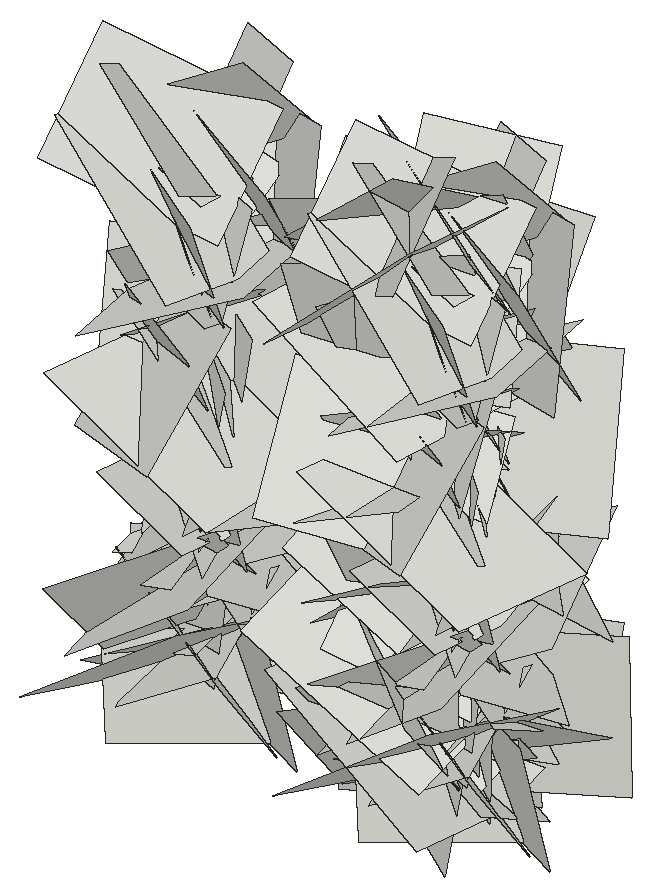
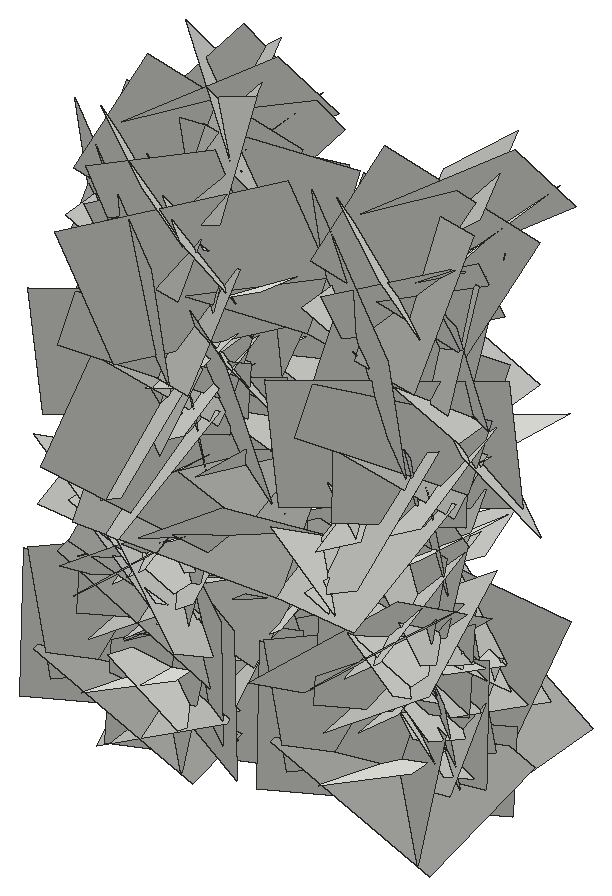
# SketchUp Ruby script. Lengths in inches.
U = 1.inch
M = Sketchup.active_model
def pt(a) = Geom::Point3d.new(a.map { |v| v * U })
def face(e, loops, mat)
  f = e.add_face(loops[0].map { |a| pt(a) })
  loops[1..].each { |l| e.add_face(l.map { |a| pt(a) }).erase! }
  f.material = f.back_material = mat if mat
  f
end
# faces: each face lists its corners as indices into pts; further lists are holes
def faces(e, pts, list, mat = nil) = list.each { |f| face(e, (f[0].is_a?(Array) ? f : [f]).map { |l| l.map { |i| pts[i] } }, mat) }
# xy, xz, yz: faces in a plane at the given z, y or x. An outline is a flat list of corners, or four numbers for a rectangle; further outlines are holes
def ring(l) = l.size == 4 ? [[l[0], l[1]], [l[2], l[1]], [l[2], l[3]], [l[0], l[3]]] : l.each_slice(2).to_a
def flat(e, list, mat, &to3) = list.each { |f| face(e, (f[0].is_a?(Array) ? f : [f]).map { |l| ring(l).map { |u, v| to3.(u, v) } }, mat) }
def xy(e, z, list, mat = nil) = flat(e, list, mat) { |x, y| [x, y, z] }
def xz(e, y, list, mat = nil) = flat(e, list, mat) { |x, z| [x, y, z] }
def yz(e, x, list, mat = nil) = flat(e, list, mat) { |y, z| [x, y, z] }
def lines(e, pts, list) = list.each { |a, b| e.add_line(pt(pts[a]), pt(pts[b])) }
# prism: a flat outline (further loops are holes) pulled along v
def prism(e, loops, v, mat = nil)
  f = face(e, loops, mat); d = Geom::Vector3d.new(v.map { |x| x * U })
  f.pushpull(f.normal.samedirection?(d) ? d.length : -d.length)
end
def box(e, o, s, mat = nil) = prism(e, [[o, [o[0] + s[0], o[1], o[2]], [o[0] + s[0], o[1] + s[1], o[2]], [o[0], o[1] + s[1], o[2]]]], [0, 0, s[2]], mat)
def at(x, y, z, deg = 0) = Geom::Transformation.translation(pt([x, y, z])) * Geom::Transformation.rotation(ORIGIN, Z_AXIS, deg.degrees)
def axes(o, x, y, z) = Geom::Transformation.new([*x, 0, *y, 0, *z, 0, *pt(o).to_a, 1])
def part(name) = M.definitions.add(name)
# library, detail: a bought-in or finely detailed component or shape, given as its bounding box
def library(name, o, s) = part(name).tap { |d| box(d.entities, o, s) }
def detail(e, o, s) = box(e.add_group.entities, o, s)
def put(e, d, t, mat = nil) = e.add_instance(d, t).tap { |i| i.material = mat if mat }
def group(e, t, mat = nil) = e.add_group.tap { |g| g.transformation = t; g.material = mat if mat }.entities
root = M.entities
c1 = part("Component\#6")
p = [[0.01,0,0],[0,3.24,4.54],[4.32,3.24,4.54],[4.33,0,0]]
faces(c1.entities,p,[[0,1,2,3]])
put(root,c1,axes([38.11,169.73,5.36],[-0.07377,0.11031,-0.61615],[-0.06228,-0.61836,-0.10407],[-0.66058,0.04598,0.07863]))
put(root,c1,axes([28.31,170.45,6.95],[0.13562,-0.59571,0.16409],[-0.06684,0.15411,0.60864],[-0.65155,-0.13981,-0.02828]))
put(root,c1,axes([34.14,170.45,6.95],[-0.13562,-0.59571,0.16409],[0.06684,0.15411,0.60864],[0.65155,-0.13981,-0.02828]))
put(root,c1,axes([38.11,170.45,6.95],[0.13562,-0.59571,0.16409],[-0.06684,0.15411,0.60864],[-0.65155,-0.13981,-0.02828]))
put(root,c1,axes([24.34,172.51,13.7],[-0.18405,-0.71312,-0.93832],[-0.0125,-0.94735,0.72216],[1.2492,-0.11455,-0.13102]))
put(root,c1,axes([38.11,172.51,13.7],[0.18405,-0.71312,-0.93832],[0.0125,-0.94735,0.72216],[-1.2492,-0.11455,-0.13102]))
put(root,c1,axes([34.14,172.51,13.7],[-0.18405,-0.71312,-0.93832],[-0.0125,-0.94735,0.72216],[1.2492,-0.11455,-0.13102]))
put(root,c1,axes([24.34,166.89,12.83],[0.13197,1.26874,-0.04114],[0.28106,-0.06642,-1.24587],[1.31589,-0.11305,0.27023]))
put(root,c1,axes([38.11,166.89,12.83],[-0.13197,1.26874,-0.04114],[-0.28106,-0.06642,-1.24587],[-1.31589,-0.11305,0.27023]))
put(root,c1,axes([34.14,166.89,12.83],[0.13197,1.26874,-0.04114],[0.28106,-0.06642,-1.24587],[1.31589,-0.11305,0.27023]))
put(root,c1,axes([28.31,170.4375,18.81],[0.19883,-0.70321,0.38228],[0.06935,0.40479,0.71252],[-0.84558,-0.13215,0.14832]))
put(root,c1,axes([34.14,170.4375,18.81],[-0.19883,-0.70321,0.38228],[-0.06935,0.40479,0.71252],[0.84558,-0.13215,0.14832]))
put(root,c1,axes([38.11,170.4375,18.81],[0.19883,-0.70321,0.38228],[0.06935,0.40479,0.71252],[-0.84558,-0.13215,0.14832]))
put(root,c1,axes([24.34,172.01,0.23],[-0.18306,-1.21621,0.26629],[-0.00588,0.26959,1.22768],[1.31971,-0.16751,0.04241]))
put(root,c1,axes([38.11,172.01,0.23],[0.18306,-1.21621,0.26629],[0.00588,0.26959,1.22768],[-1.31971,-0.16751,0.04241]))
put(root,c1,axes([34.14,172.01,0.23],[-0.18306,-1.21621,0.26629],[-0.00588,0.26959,1.22768],[1.31971,-0.16751,0.04241]))
put(root,c1,axes([24.34,167.43,21.54],[0.05686,1.16606,-0.16138],[-0.18622,-0.15181,-1.15529],[1.23383,-0.07665,-0.16693]))
put(root,c1,axes([38.11,167.43,21.54],[-0.05686,1.16606,-0.16138],[0.18622,-0.15181,-1.15529],[-1.23383,-0.07665,-0.16693]))
put(root,c1,axes([34.14,167.43,21.54],[0.05686,1.16606,-0.16138],[-0.18622,-0.15181,-1.15529],[1.23383,-0.07665,-0.16693]))
put(root,c1,axes([24.34,170.29,20.28],[0.01759,0.35165,-0.94572],[0.09141,-0.94289,-0.34909],[1.06561,0.07508,0.04555]))
put(root,c1,axes([38.11,170.29,20.28],[-0.01759,0.35165,-0.94572],[-0.09141,-0.94289,-0.34909],[-1.06561,0.07508,0.04555]))
put(root,c1,axes([34.14,170.29,20.28],[0.01759,0.35165,-0.94572],[0.09141,-0.94289,-0.34909],[1.06561,0.07508,0.04555]))
put(root,c1,axes([24.34,166.61,20.4],[0.01588,0.7114,0.79833],[-0.18087,0.78977,-0.70057],[1.11894,0.11757,-0.12458]))
put(root,c1,axes([38.11,166.61,20.4],[-0.01588,0.7114,0.79833],[0.18087,0.78977,-0.70057],[-1.11894,0.11757,-0.12458]))
put(root,c1,axes([34.14,166.61,20.4],[0.01588,0.7114,0.79833],[-0.18087,0.78977,-0.70057],[1.11894,0.11757,-0.12458]))
put(root,c1,axes([28.31,169.875,11.58],[0.08121,-0.31714,0.54408],[-0.11401,0.53345,0.32609],[-0.65774,-0.13162,0.01065]))
put(root,c1,axes([34.14,169.875,11.58],[-0.08121,-0.31714,0.54408],[0.11401,0.53345,0.32609],[0.65774,-0.13162,0.01065]))
put(root,c1,axes([38.11,169.875,11.58],[0.08121,-0.31714,0.54408],[-0.11401,0.53345,0.32609],[-0.65774,-0.13162,0.01065]))
put(root,c1,axes([24.34,169.82,1.95],[-0.02915,-0.64251,0.76006],[-0.08177,0.75943,0.6392],[1.05178,0.04123,0.07076]))
put(root,c1,axes([38.11,169.82,1.95],[0.02915,-0.64251,0.76006],[0.08177,0.75943,0.6392],[-1.05178,0.04123,0.07076]))
put(root,c1,axes([34.14,169.82,1.95],[-0.02915,-0.64251,0.76006],[-0.08177,0.75943,0.6392],[1.05178,0.04123,0.07076]))
put(root,c1,axes([24.34,173.1,4.27],[0.006,-1.20261,-0.38975],[-0.07836,-0.3894,1.20046],[1.33775,-0.01742,0.07206]))
put(root,c1,axes([38.11,173.1,4.27],[-0.006,-1.20261,-0.38975],[0.07836,-0.3894,1.20046],[-1.33775,-0.01742,0.07206]))
put(root,c1,axes([34.14,173.1,4.27],[0.006,-1.20261,-0.38975],[-0.07836,-0.3894,1.20046],[1.33775,-0.01742,0.07206]))
put(root,c1,axes([28.31,169.57,7.53],[-0.02893,-0.34038,0.60393],[0.06424,0.60091,0.34142],[-0.73203,0.06619,0.00609]))
put(root,c1,axes([34.14,169.57,7.53],[0.02893,-0.34038,0.60393],[-0.06424,0.60091,0.34142],[0.73203,0.06619,0.00609]))
put(root,c1,axes([38.11,169.57,7.53],[-0.02893,-0.34038,0.60393],[0.06424,0.60091,0.34142],[-0.73203,0.06619,0.00609]))
put(root,c1,axes([24.34,172.68,14.25],[0.15371,-1.16437,-0.05617],[0.14183,-0.0396,1.1664],[1.22751,0.15038,-0.12774]))
put(root,c1,axes([38.11,172.68,14.25],[-0.15371,-1.16437,-0.05617],[-0.14183,-0.0396,1.1664],[-1.22751,0.15038,-0.12774]))
put(root,c1,axes([34.14,172.68,14.25],[0.15371,-1.16437,-0.05617],[0.14183,-0.0396,1.1664],[1.22751,0.15038,-0.12774]))
put(root,c1,axes([28.31,172.08,18.68],[0.05145,-0.65016,0.07549],[-0.09383,0.06848,0.64671],[-0.68743,-0.05801,-0.08262]))
put(root,c1,axes([38.11,172.08,18.68],[0.05145,-0.65016,0.07549],[-0.09383,0.06848,0.64671],[-0.68743,-0.05801,-0.08262]))
put(root,c1,axes([34.14,172.08,18.68],[-0.05145,-0.65016,0.07549],[0.09383,0.06848,0.64671],[0.68743,-0.05801,-0.08262]))
put(root,c1,axes([28.31,168.08,6.15],[0.10311,0.69666,0.5447],[0.01855,0.54636,-0.70191],[-0.9372,0.08746,0.04604]))
put(root,c1,axes([34.14,168.08,6.15],[-0.10311,0.69666,0.5447],[-0.01855,0.54636,-0.70191],[0.9372,0.08746,0.04604]))
put(root,c1,axes([38.11,168.08,6.15],[0.10311,0.69666,0.5447],[0.01855,0.54636,-0.70191],[-0.9372,0.08746,0.04604]))
put(root,c1,axes([24.34,170.37,5.28],[-0.04044,0.69271,-0.86885],[0.14808,-0.85947,-0.69137],[1.16852,0.13289,0.05755]))
put(root,c1,axes([38.11,170.37,5.28],[0.04044,0.69271,-0.86885],[-0.14808,-0.85947,-0.69137],[-1.16852,0.13289,0.05755]))
put(root,c1,axes([34.14,170.37,5.28],[-0.04044,0.69271,-0.86885],[0.14808,-0.85947,-0.69137],[1.16852,0.13289,0.05755]))
put(root,c1,axes([24.34,171.61,19.65],[-0.05512,0.44879,-0.89687],[-0.12411,-0.89465,-0.44089],[1.05579,-0.08174,-0.09865]))
put(root,c1,axes([38.11,171.61,19.65],[0.05512,0.44879,-0.89687],[0.12411,-0.89465,-0.44089],[-1.05579,-0.08174,-0.09865]))
put(root,c1,axes([34.14,171.61,19.65],[-0.05512,0.44879,-0.89687],[-0.12411,-0.89465,-0.44089],[1.05579,-0.08174,-0.09865]))
put(root,c1,axes([24.34,172.8125,18.6875],[-0.10377,-0.25363,-0.96814],[0.17625,-0.96337,0.23557],[1.04612,0.13715,-0.13572]))
put(root,c1,axes([38.11,172.8125,18.6875],[0.10377,-0.25363,-0.96814],[-0.17625,-0.96337,0.23557],[-1.04612,0.13715,-0.13572]))
put(root,c1,axes([34.14,172.8125,18.6875],[-0.10377,-0.25363,-0.96814],[0.17625,-0.96337,0.23557],[1.04612,0.13715,-0.13572]))
put(root,c1,axes([24.34,173.43,2.26],[0.13173,-0.86629,-0.47025],[-0.00519,-0.47451,0.87284],[1.04483,0.10686,0.06363]))
put(root,c1,axes([38.11,173.43,2.26],[-0.13173,-0.86629,-0.47025],[0.00519,-0.47451,0.87284],[-1.04483,0.10686,0.06363]))
put(root,c1,axes([34.14,173.43,2.26],[0.13173,-0.86629,-0.47025],[-0.00519,-0.47451,0.87284],[1.04483,0.10686,0.06363]))
put(root,c1,axes([28.31,172.62,2.82],[0.11022,-0.07985,-0.84847],[-0.01268,-0.85481,0.07898],[-0.90326,0.00226,-0.10464]))
put(root,c1,axes([34.14,172.62,2.82],[-0.11022,-0.07985,-0.84847],[0.01268,-0.85481,0.07898],[0.90326,0.00226,-0.10464]))
put(root,c1,axes([38.11,172.62,2.82],[0.11022,-0.07985,-0.84847],[-0.01268,-0.85481,0.07898],[-0.90326,0.00226,-0.10464]))
put(root,c1,axes([38.11,172.18,10.26],[-0.13568,0.14362,-0.9313],[-0.0793,-0.93844,-0.13444],[-0.9957,0.05517,0.13761]))
put(root,c1,axes([24.34,172.18,10.26],[0.13568,0.14362,-0.9313],[0.0793,-0.93844,-0.13444],[0.9957,0.05517,0.13761]))
put(root,c1,axes([34.14,172.18,10.26],[0.13568,0.14362,-0.9313],[0.0793,-0.93844,-0.13444],[0.9957,0.05517,0.13761]))
put(root,c1,axes([28.31,169.25,3.37],[0.12984,0.58451,0.34416],[0.01188,0.34794,-0.59491],[-0.71891,0.11132,0.05233]))
put(root,c1,axes([34.14,169.25,3.37],[-0.12984,0.58451,0.34416],[-0.01188,0.34794,-0.59491],[0.71891,0.11132,0.05233]))
put(root,c1,axes([38.11,169.25,3.37],[0.12984,0.58451,0.34416],[0.01188,0.34794,-0.59491],[-0.71891,0.11132,0.05233]))
put(root,c1,axes([24.34,174.625,6.88],[0.07025,-1.10898,-0.49527],[-0.16839,-0.49966,1.09755],[1.27636,-0.00489,0.17206]))
put(root,c1,axes([38.11,174.625,6.88],[-0.07025,-1.10898,-0.49527],[0.16839,-0.49966,1.09755],[-1.27636,-0.00489,0.17206]))
put(root,c1,axes([34.14,174.625,6.88],[0.07025,-1.10898,-0.49527],[-0.16839,-0.49966,1.09755],[1.27636,-0.00489,0.17206]))
put(root,c1,axes([24.34,173.47,4.9],[0.07332,-0.2848,-0.87141],[-0.0336,-0.87411,0.28317],[0.9712,-0.00874,0.07558]))
put(root,c1,axes([38.11,173.47,4.9],[-0.07332,-0.2848,-0.87141],[0.0336,-0.87411,0.28317],[-0.9712,-0.00874,0.07558]))
put(root,c1,axes([34.14,173.47,4.9],[0.07332,-0.2848,-0.87141],[-0.0336,-0.87411,0.28317],[0.9712,-0.00874,0.07558]))
put(root,c1,axes([28.31,169.67,8.54],[0.12628,0.08221,0.86907],[0.11161,0.86937,-0.09667],[-0.91857,0.11693,0.10773]))
put(root,c1,axes([34.14,169.67,8.54],[-0.12628,0.08221,0.86907],[-0.11161,0.86937,-0.09667],[0.91857,0.11693,0.10773]))
put(root,c1,axes([38.11,169.67,8.54],[0.12628,0.08221,0.86907],[0.11161,0.86937,-0.09667],[-0.91857,0.11693,0.10773]))
put(root,c1,axes([28.31,173.61,18.42],[-0.00387,-0.64214,-0.38262],[-0.01033,-0.38255,0.64212],[-0.79227,0.00812,-0.0065]))
put(root,c1,axes([34.14,173.61,18.42],[0.00387,-0.64214,-0.38262],[0.01033,-0.38255,0.64212],[0.79227,0.00812,-0.0065]))
put(root,c1,axes([38.11,173.61,18.42],[-0.00387,-0.64214,-0.38262],[-0.01033,-0.38255,0.64212],[-0.79227,0.00812,-0.0065]))
put(root,c1,axes([24.34,173.47,6.03],[-0.02519,-0.71274,-0.22366],[0.1783,-0.22314,0.69319],[0.7715,0.02829,-0.1675]))
put(root,c1,axes([38.11,173.47,6.03],[0.02519,-0.71274,-0.22366],[-0.1783,-0.22314,0.69319],[-0.7715,0.02829,-0.1675]))
put(root,c1,axes([34.14,173.47,6.03],[-0.02519,-0.71274,-0.22366],[0.1783,-0.22314,0.69319],[0.7715,0.02829,-0.1675]))
put(root,c1,axes([24.34,170.23,14.27],[-0.02775,1.05616,-0.50439],[-0.01222,-0.50473,-1.05626],[1.24058,0.01865,-0.02169]))
put(root,c1,axes([38.11,170.23,14.27],[0.02775,1.05616,-0.50439],[0.01222,-0.50473,-1.05626],[-1.24058,0.01865,-0.02169]))
put(root,c1,axes([34.14,170.23,14.27],[-0.02775,1.05616,-0.50439],[-0.01222,-0.50473,-1.05626],[1.24058,0.01865,-0.02169]))
put(root,c1,axes([24.34,172.3,17.31],[-0.17712,-0.66279,0.75583],[0.05377,0.75967,0.67737],[1.06423,-0.14869,0.09157]))
put(root,c1,axes([38.11,172.3,17.31],[0.17712,-0.66279,0.75583],[-0.05377,0.75967,0.67737],[-1.06423,-0.14869,0.09157]))
put(root,c1,axes([34.14,172.3,17.31],[-0.17712,-0.66279,0.75583],[0.05377,0.75967,0.67737],[1.06423,-0.14869,0.09157]))
put(root,c1,axes([24.34,171.9,21.66],[0.05821,0.63814,-1.10333],[0.23209,-1.09266,-0.62107],[1.33097,0.16262,0.15656]))
put(root,c1,axes([38.11,171.9,21.66],[-0.05821,0.63814,-1.10333],[-0.23209,-1.09266,-0.62107],[-1.33097,0.16262,0.15656]))
put(root,c1,axes([34.14,171.9,21.66],[0.05821,0.63814,-1.10333],[0.23209,-1.09266,-0.62107],[1.33097,0.16262,0.15656]))
put(root,c1,axes([28.31,171.64,6.09],[0.04085,-0.22846,0.61977],[-0.06336,0.61707,0.23119],[-0.6973,-0.06945,0.0153]))
put(root,c1,axes([34.14,171.64,6.09],[-0.04085,-0.22846,0.61977],[0.06336,0.61707,0.23119],[0.6973,-0.06945,0.0153]))
put(root,c1,axes([38.11,171.64,6.09],[0.04085,-0.22846,0.61977],[-0.06336,0.61707,0.23119],[-0.6973,-0.06945,0.0153]))
put(root,c1,axes([24.34,170.14,10.52],[0.06349,0.95893,0.01002],[-0.03302,0.01198,-0.96028],[1.01599,-0.05954,-0.03183]))
put(root,c1,axes([38.11,170.14,10.52],[-0.06349,0.95893,0.01002],[0.03302,0.01198,-0.96028],[-1.01599,-0.05954,-0.03183]))
put(root,c1,axes([34.14,170.14,10.52],[0.06349,0.95893,0.01002],[-0.03302,0.01198,-0.96028],[1.01599,-0.05954,-0.03183]))
put(root,c1,axes([28.31,174.87,19.3],[0.1513,-0.51657,-0.73784],[0.06675,-0.7395,0.52991],[-0.9524,-0.13389,-0.08008]))
put(root,c1,axes([34.14,174.87,19.3],[-0.1513,-0.51657,-0.73784],[-0.06675,-0.7395,0.52991],[0.9524,-0.13389,-0.08008]))
put(root,c1,axes([38.11,174.87,19.3],[0.1513,-0.51657,-0.73784],[0.06675,-0.7395,0.52991],[-0.9524,-0.13389,-0.08008]))
put(root,c1,axes([24.34,172.92,11.6],[0.15777,-0.72106,0.34948],[-0.01112,0.35368,0.73418],[0.84929,0.13857,-0.05531]))
put(root,c1,axes([38.11,172.92,11.6],[-0.15777,-0.72106,0.34948],[0.01112,0.35368,0.73418],[-0.84929,0.13857,-0.05531]))
put(root,c1,axes([34.14,172.92,11.6],[0.15777,-0.72106,0.34948],[-0.01112,0.35368,0.73418],[0.84929,0.13857,-0.05531]))
put(root,c1,axes([24.34,169.35,10.4],[-0.15861,0.37048,1.309],[0.06067,1.31744,-0.36632],[1.44077,-0.01469,0.15953]))
put(root,c1,axes([38.11,169.35,10.4],[0.15861,0.37048,1.309],[-0.06067,1.31744,-0.36632],[-1.44077,-0.01469,0.15953]))
put(root,c1,axes([34.14,169.35,10.4],[-0.15861,0.37048,1.309],[0.06067,1.31744,-0.36632],[1.44077,-0.01469,0.15953]))
put(root,c1,axes([24.34,171.5,10.51],[0.09816,1.08592,-0.68794],[-0.27584,-0.65961,-1.07622],[1.33441,-0.21623,-0.17187]))
put(root,c1,axes([38.11,171.5,10.51],[-0.09816,1.08592,-0.68794],[0.27584,-0.65961,-1.07622],[-1.33441,-0.21623,-0.17187]))
put(root,c1,axes([34.14,171.5,10.51],[0.09816,1.08592,-0.68794],[-0.27584,-0.65961,-1.07622],[1.33441,-0.21623,-0.17187]))
put(root,c1,axes([24.34,170.67,8.7],[-0.18467,1.04701,-0.56036],[-0.0341,-0.57031,-1.0556],[1.25832,0.1382,-0.11085]))
put(root,c1,axes([38.11,170.67,8.7],[0.18467,1.04701,-0.56036],[0.0341,-0.57031,-1.0556],[-1.25832,0.1382,-0.11085]))
put(root,c1,axes([34.14,170.67,8.7],[-0.18467,1.04701,-0.56036],[-0.0341,-0.57031,-1.0556],[1.25832,0.1382,-0.11085]))
put(root,c1,axes([24.34,174.22,3.89],[0.08779,-0.72671,-0.31501],[0.02258,-0.31457,0.73129],[0.83927,0.08448,0.01327]))
put(root,c1,axes([38.11,174.22,3.89],[-0.08779,-0.72671,-0.31501],[-0.02258,-0.31457,0.73129],[-0.83927,0.08448,0.01327]))
put(root,c1,axes([34.14,174.22,3.89],[0.08779,-0.72671,-0.31501],[0.02258,-0.31457,0.73129],[0.83927,0.08448,0.01327]))
put(root,c1,axes([24.34,174.19,-1.125],[-0.19779,-1.01545,0.55728],[0.13113,0.54376,1.03224],[1.22079,-0.22293,-0.02059]))
put(root,c1,axes([38.11,174.19,-1.125],[0.19779,-1.01545,0.55728],[-0.13113,0.54376,1.03224],[-1.22079,-0.22293,-0.02059]))
put(root,c1,axes([34.14,174.19,-1.125],[-0.19779,-1.01545,0.55728],[0.13113,0.54376,1.03224],[1.22079,-0.22293,-0.02059]))
put(root,c1,axes([28.31,171.41,10.85],[0.07762,0.04197,0.59758],[-0.0194,0.6019,-0.04003],[-0.6347,-0.01326,0.07431]))
put(root,c1,axes([34.14,171.41,10.85],[-0.07762,0.04197,0.59758],[0.0194,0.6019,-0.04003],[0.6347,-0.01326,0.07431]))
put(root,c1,axes([38.11,171.41,10.85],[0.07762,0.04197,0.59758],[-0.0194,0.6019,-0.04003],[-0.6347,-0.01326,0.07431]))
put(root,c1,axes([24.34,173.32,3.72],[0.0912,0.22313,-1.04907],[0.17676,-1.04242,-0.20804],[1.12306,0.14594,0.11794]))
put(root,c1,axes([38.11,173.32,3.72],[-0.0912,0.22313,-1.04907],[-0.17676,-1.04242,-0.20804],[-1.12306,0.14594,0.11794]))
put(root,c1,axes([34.14,173.32,3.72],[0.0912,0.22313,-1.04907],[0.17676,-1.04242,-0.20804],[1.12306,0.14594,0.11794]))
put(root,c1,axes([28.31,173.27,2.31],[-0.02745,-0.60704,0.2793],[0.09658,0.2737,0.6033],[-0.70169,0.06142,0.07211]))
put(root,c1,axes([34.14,173.27,2.31],[0.02745,-0.60704,0.2793],[-0.09658,0.2737,0.6033],[0.70169,0.06142,0.07211]))
put(root,c1,axes([38.11,173.27,2.31],[-0.02745,-0.60704,0.2793],[0.09658,0.2737,0.6033],[-0.70169,0.06142,0.07211]))
put(root,c1,axes([24.34,172.23,12.17],[0.04321,-0.56467,0.8488],[-0.06772,0.84639,0.56613],[1.07851,0.07577,0.00154]))
put(root,c1,axes([38.11,172.23,12.17],[-0.04321,-0.56467,0.8488],[0.06772,0.84639,0.56613],[-1.07851,0.07577,0.00154]))
put(root,c1,axes([34.14,172.23,12.17],[0.04321,-0.56467,0.8488],[-0.06772,0.84639,0.56613],[1.07851,0.07577,0.00154]))
put(root,c1,axes([24.34,170.77,1.94],[0.10305,0.14958,1.1623],[-0.03,1.16625,-0.14772],[1.24184,0.01576,-0.10002]))
put(root,c1,axes([38.11,170.77,1.94],[-0.10305,0.14958,1.1623],[0.03,1.16625,-0.14772],[-1.24184,0.01576,-0.10002]))
put(root,c1,axes([34.14,170.77,1.94],[0.10305,0.14958,1.1623],[-0.03,1.16625,-0.14772],[1.24184,0.01576,-0.10002]))
put(root,c1,axes([24.34,172.28,10.96],[0.19399,-0.26613,0.68464],[-0.06344,0.69782,0.28725],[0.77602,0.12358,-0.14766]))
put(root,c1,axes([38.11,172.28,10.96],[-0.19399,-0.26613,0.68464],[0.06344,0.69782,0.28725],[-0.77602,0.12358,-0.14766]))
put(root,c1,axes([34.14,172.28,10.96],[0.19399,-0.26613,0.68464],[-0.06344,0.69782,0.28725],[0.77602,0.12358,-0.14766]))
put(root,c1,axes([24.34,172.17,3.88],[0.10658,-0.21665,0.83392],[-0.00523,0.83942,0.21867],[0.91328,0.03009,-0.09606]))
put(root,c1,axes([38.11,172.17,3.88],[-0.10658,-0.21665,0.83392],[0.00523,0.83942,0.21867],[-0.91328,0.03009,-0.09606]))
put(root,c1,axes([34.14,172.17,3.88],[0.10658,-0.21665,0.83392],[-0.00523,0.83942,0.21867],[0.91328,0.03009,-0.09606]))
put(root,c1,axes([24.34,172.79,12.08],[0.24348,0.91998,-0.78066],[0.03668,-0.79938,-0.93185],[1.27843,-0.15228,0.17542]))
put(root,c1,axes([38.11,172.79,12.08],[-0.24348,0.91998,-0.78066],[-0.03668,-0.79938,-0.93185],[-1.27843,-0.15228,0.17542]))
put(root,c1,axes([34.14,172.79,12.08],[0.24348,0.91998,-0.78066],[0.03668,-0.79938,-0.93185],[1.27843,-0.15228,0.17542]))
put(root,c1,axes([38.11,171.28,0.09],[0.0277,-0.00252,1.28462],[-0.09278,1.2819,0.0043],[-1.35854,-0.08759,0.0259]))
put(root,c1,axes([24.34,171.28,0.09],[-0.0277,-0.00252,1.28462],[0.09278,1.2819,0.0043],[1.35854,-0.08759,0.0259]))
put(root,c1,axes([34.14,171.28,0.09],[-0.0277,-0.00252,1.28462],[0.09278,1.2819,0.0043],[1.35854,-0.08759,0.0259]))
put(root,c1,axes([28.31,174.97,1.18],[0.10067,-0.62121,-0.06126],[-0.13552,-0.08001,0.61313],[-0.64765,-0.07982,-0.13782]))
put(root,c1,axes([34.14,174.97,1.18],[-0.10067,-0.62121,-0.06126],[0.13552,-0.08001,0.61313],[0.64765,-0.07982,-0.13782]))
put(root,c1,axes([38.11,174.97,1.18],[0.10067,-0.62121,-0.06126],[-0.13552,-0.08001,0.61313],[-0.64765,-0.07982,-0.13782]))
put(root,c1,axes([24.34,176.36,18.92],[0.19548,-0.4632,-1.27504],[-0.04093,-1.28804,0.46234],[1.43738,0.02631,0.18657]))
put(root,c1,axes([38.11,176.36,18.92],[-0.19548,-0.4632,-1.27504],[0.04093,-1.28804,0.46234],[-1.43738,0.02631,0.18657]))
put(root,c1,axes([34.14,176.36,18.92],[0.19548,-0.4632,-1.27504],[-0.04093,-1.28804,0.46234],[1.43738,0.02631,0.18657]))
put(root,c1,axes([24.34,176.11,6.43],[0.23133,-1.0261,-0.61864],[0.04368,-0.62202,1.04624],[1.2693,0.20842,0.07674]))
put(root,c1,axes([38.11,176.11,6.43],[-0.23133,-1.0261,-0.61864],[-0.04368,-0.62202,1.04624],[-1.2693,0.20842,0.07674]))
put(root,c1,axes([34.14,176.11,6.43],[0.23133,-1.0261,-0.61864],[0.04368,-0.62202,1.04624],[1.2693,0.20842,0.07674]))
put(root,c1,axes([24.34,175.17,6.35],[0.11089,-0.78923,-0.08985],[0.10937,-0.07636,0.79084],[0.83485,0.11483,-0.09167]))
put(root,c1,axes([38.11,175.17,6.35],[-0.11089,-0.78923,-0.08985],[-0.10937,-0.07636,0.79084],[-0.83485,0.11483,-0.09167]))
put(root,c1,axes([34.14,175.17,6.35],[0.11089,-0.78923,-0.08985],[0.10937,-0.07636,0.79084],[0.83485,0.11483,-0.09167]))
put(root,c1,axes([28.31,175.4,4.97],[-0.01432,-0.74639,-0.04739],[0.08616,-0.04858,0.74199],[-0.78807,0.00825,0.08199]))
put(root,c1,axes([34.14,175.4,4.97],[0.01432,-0.74639,-0.04739],[-0.08616,-0.04858,0.74199],[0.78807,0.00825,0.08199]))
put(root,c1,axes([38.11,175.4,4.97],[-0.01432,-0.74639,-0.04739],[0.08616,-0.04858,0.74199],[-0.78807,0.00825,0.08199]))
put(root,c1,axes([24.34,173.68,14.42],[0.07839,0.88361,-0.83437],[-0.27617,-0.80495,-0.87555],[1.25826,-0.23172,-0.14019]))
put(root,c1,axes([38.11,173.68,14.42],[-0.07839,0.88361,-0.83437],[0.27617,-0.80495,-0.87555],[-1.25826,-0.23172,-0.14019]))
put(root,c1,axes([34.14,173.68,14.42],[0.07839,0.88361,-0.83437],[-0.27617,-0.80495,-0.87555],[1.25826,-0.23172,-0.14019]))
put(root,c1,axes([28.31,171.94,19.49],[0.08782,0.36838,0.63269],[-0.00702,0.63708,-0.37006],[-0.77601,0.03592,0.07495]))
put(root,c1,axes([34.14,171.94,19.49],[-0.08782,0.36838,0.63269],[0.00702,0.63708,-0.37006],[0.77601,0.03592,0.07495]))
put(root,c1,axes([38.11,171.94,19.49],[0.08782,0.36838,0.63269],[-0.00702,0.63708,-0.37006],[-0.77601,0.03592,0.07495]))
put(root,c1,axes([24.34,170.9375,7.01],[0.11124,0.9843,0.53665],[-0.15751,0.54645,-0.97322],[1.17787,-0.01989,-0.18083]))
put(root,c1,axes([38.11,170.9375,7.01],[-0.11124,0.9843,0.53665],[0.15751,0.54645,-0.97322],[-1.17787,-0.01989,-0.18083]))
